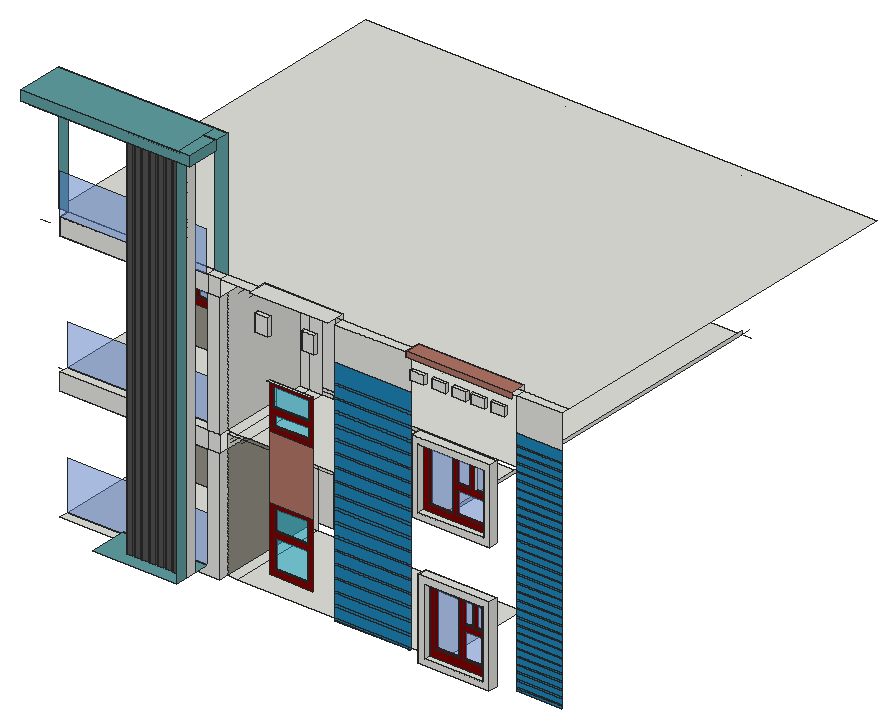
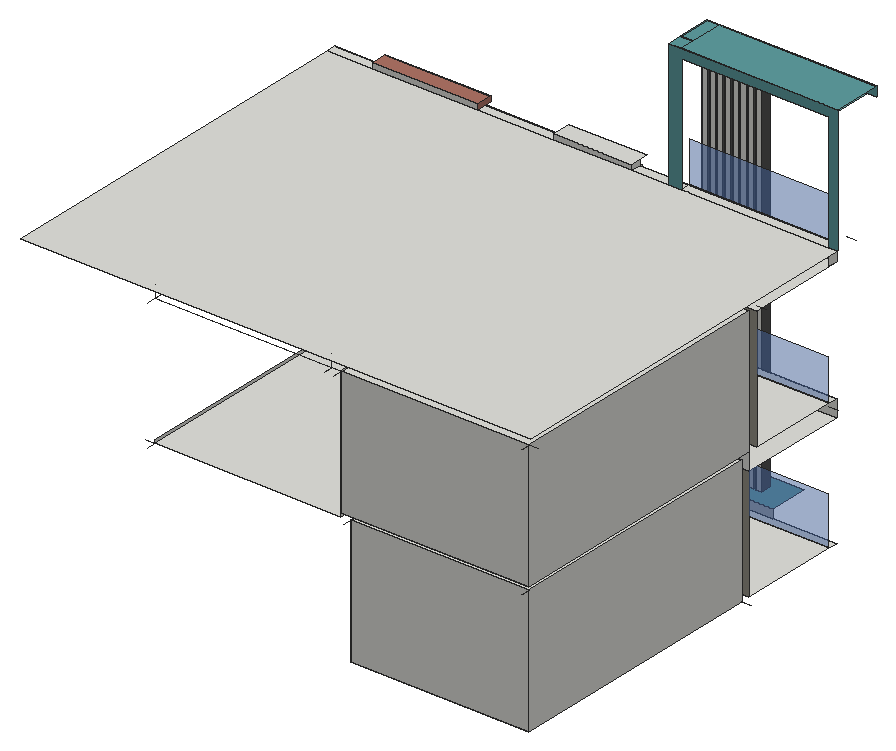
# SketchUp Ruby script. Lengths in inches.
U = 1.inch
M = Sketchup.active_model
def pt(a) = Geom::Point3d.new(a.map { |v| v * U })
def face(e, loops, mat)
  f = e.add_face(loops[0].map { |a| pt(a) })
  loops[1..].each { |l| e.add_face(l.map { |a| pt(a) }).erase! }
  f.material = f.back_material = mat if mat
  f
end
# faces: each face lists its corners as indices into pts; further lists are holes
def faces(e, pts, list, mat = nil) = list.each { |f| face(e, (f[0].is_a?(Array) ? f : [f]).map { |l| l.map { |i| pts[i] } }, mat) }
# xy, xz, yz: faces in a plane at the given z, y or x. An outline is a flat list of corners, or four numbers for a rectangle; further outlines are holes
def ring(l) = l.size == 4 ? [[l[0], l[1]], [l[2], l[1]], [l[2], l[3]], [l[0], l[3]]] : l.each_slice(2).to_a
def flat(e, list, mat, &to3) = list.each { |f| face(e, (f[0].is_a?(Array) ? f : [f]).map { |l| ring(l).map { |u, v| to3.(u, v) } }, mat) }
def xy(e, z, list, mat = nil) = flat(e, list, mat) { |x, y| [x, y, z] }
def xz(e, y, list, mat = nil) = flat(e, list, mat) { |x, z| [x, y, z] }
def yz(e, x, list, mat = nil) = flat(e, list, mat) { |y, z| [x, y, z] }
def lines(e, pts, list) = list.each { |a, b| e.add_line(pt(pts[a]), pt(pts[b])) }
# prism: a flat outline (further loops are holes) pulled along v
def prism(e, loops, v, mat = nil)
  f = face(e, loops, mat); d = Geom::Vector3d.new(v.map { |x| x * U })
  f.pushpull(f.normal.samedirection?(d) ? d.length : -d.length)
end
def box(e, o, s, mat = nil) = prism(e, [[o, [o[0] + s[0], o[1], o[2]], [o[0] + s[0], o[1] + s[1], o[2]], [o[0], o[1] + s[1], o[2]]]], [0, 0, s[2]], mat)
def at(x, y, z, deg = 0) = Geom::Transformation.translation(pt([x, y, z])) * Geom::Transformation.rotation(ORIGIN, Z_AXIS, deg.degrees)
def axes(o, x, y, z) = Geom::Transformation.new([*x, 0, *y, 0, *z, 0, *pt(o).to_a, 1])
def part(name) = M.definitions.add(name)
# library, detail: a bought-in or finely detailed component or shape, given as its bounding box
def library(name, o, s) = part(name).tap { |d| box(d.entities, o, s) }
def detail(e, o, s) = box(e.add_group.entities, o, s)
def put(e, d, t, mat = nil) = e.add_instance(d, t).tap { |i| i.material = mat if mat }
def group(e, t, mat = nil) = e.add_group.tap { |g| g.transformation = t; g.material = mat if mat }.entities
root = M.entities
M.materials.add("[0022_Maroon]").color = [128, 0, 0]
M.materials.add("[0081_CadetBlue]").color = [95, 158, 160]
M.materials.add("[0100_SteelBlue]").color = [29, 130, 180]
M.materials.add("[0135_DarkGray]").color = [81, 81, 81]
M.materials.add("[Formica Graystone]").color = [149, 146, 135]
M.materials.add("[Stone Flagstone Ashlar]").color = [175, 116, 102]
M.materials.add("[Translucent Glass Blue]").color = [100, 149, 237]
M.materials["[Translucent Glass Blue]"].alpha = 0.5
M.materials.add("[Translucent Glass Tinted]").color = [8, 201, 241]
M.materials["[Translucent Glass Tinted]"].alpha = 0.48
box(root,[9,148.25,428.75],[169.01,251.0625,120])
xy(root,428.75,[[9,36,160.01,45],[9,45,160.01,45,160.01,139.25,141.38,139.25,141.38,136.25,138.38,136.25,138.38,139.25,102.38,139.25,102.38,136.25,99.38,136.25,99.38,139.25,9,139.25],[160.01,45,170.26,139.25],[170.26,45,363.3125,139.25],[99.38,136.25,102.38,139.25],
  [138.38,136.25,141.38,139.25]])
xy(root,434.83,[[359.73,21,427.1,30]])
xy(root,437.26,[[[69.02,0,148.21,0,148.21,12,142.39,12,142.39,21.4,148.21,21.4,148.21,36,69.02,36],[98.52,12,98.52,21.4,104.33,21.4,104.33,12,105.83,12,105.83,21.4,111.64,21.4,111.64,12],[91.21,12,97.02,21.4],[127.77,12,133.58,21.4],[135.08,12,140.89,21.4]]],"[0081_CadetBlue]")
xy(root,437.3,[[113.14,12,118.96,21.4],[120.46,12,126.27,21.4]])
xy(root,440.83,[[365.73,21,421.1,27],[365.73,27,421.1,30]])
xy(root,447.86,[[371.08,27,393.35,30],[398.07,27,415.61,30]],"[0022_Maroon]")
xy(root,459.79,[[217.16,30,247.77,31.875]],"[0022_Maroon]")
xy(root,473.34,[[19,136.25,77.07,139.25]])
xy(root,473.35,[[398.07,27,415.61,30]],"[0022_Maroon]")
xy(root,477.84,[[398.07,27,406.84,30],[408.875,27,415.61,30]],"[0022_Maroon]")
xy(root,479.34,[[25,136.25,43.41,139.25],[48.03,136.25,71.07,139.25]],"[0022_Maroon]")
xy(root,486.74,[[217.16,30,247.77,31.875]],"[0022_Maroon]")
xy(root,492.12,[[217.16,30,247.77,32.25]],"[0022_Maroon]")
xy(root,498.84,[[371.08,27,393.35,30],[398.07,27,406.84,30],[408.875,27,415.61,30]],"[0022_Maroon]")
xy(root,504.21,[[365.73,21,421.1,27],[365.73,27,421.1,30]])
xy(root,504.65,[[48.03,136.25,71.07,139.25]],"[0022_Maroon]")
xy(root,508.1,[[48.03,136.25,71.07,139.25]],"[0022_Maroon]")
xy(root,510.21,[[359.73,21,427.1,30]])
xy(root,511.875,[[217.16,30,247.77,32.25]],"[0022_Maroon]")
xy(root,512.75,[[102.38,136.25,138.38,139.25]])
xy(root,515.75,[[99.38,136.25,141.38,139.25]])
xy(root,520.4,[[25,136.25,43.41,139.25],[48.03,136.25,71.07,139.25]],"[0022_Maroon]")
xy(root,526.4,[[19,136.25,77.07,139.25]])
xy(root,535.625,[[9,36,160.01,139.25]])
xy(root,548.75,[[160.01,45,170.26,139.25],[187.01,139.25,363.3125,399.3125]])
xy(root,551.75,[[9,36,160.01,45],[9,45,160.01,130.25],[160.01,45,170.26,130.25],[170.26,45,180.76,130.25],[180.76,45,363.3125,130.25],
  [9,139.25,187.01,399.3125]])
xy(root,556.6,[[353.5625,21,427.4375,30]])
xy(root,562.6,[[359.5625,21,421.4375,27]])
xy(root,568.2,[[365.03,27,387.7,30],[391.2,27,417.37,30]],"[0022_Maroon]")
xy(root,580.49,[[215.47,30,248.72,32.875]],"[0022_Maroon]")
xy(root,589.01,[[28.48,127.25,94.79,130.25]])
xy(root,590.47,[[391.2,27,417.37,30]],"[0022_Maroon]")
xy(root,591.16,[[215.47,30,248.72,32.875]],"[0022_Maroon]")
xy(root,595.01,[[34.48,127.25,61.63,130.25],[65.6,127.25,88.79,130.25]],"[0022_Maroon]")
xy(root,595.1,[[391.2,27,404.29,30],[408.3,27,417.37,30]],"[0022_Maroon]")
xy(root,596.41,[[215.47,32.3125,248.72,33.5]])
xy(root,596.47,[[215.47,30,248.72,32.3125]],"[0022_Maroon]")
xy(root,614.66,[[215.47,32.3125,248.72,33.5]])
xy(root,614.66,[[215.47,30,248.72,32.3125]],"[0022_Maroon]")
xy(root,616.91,[[365.03,27,387.7,30],[391.2,27,404.29,30],[408.3,27,417.37,30]],"[0022_Maroon]")
xy(root,619.47,[[211.91,27,253.16,30]])
xy(root,620.6,[[359.5625,21,421.4375,27]])
xy(root,626.6,[[353.5625,21,427.4375,30]])
xy(root,630.26,[[65.6,127.25,88.79,130.25]],"[0022_Maroon]")
xy(root,635.12,[[65.6,127.25,88.79,130.25]],"[0022_Maroon]")
xy(root,649.32,[[34.48,127.25,61.63,130.25],[65.6,127.25,88.79,130.25]],"[0022_Maroon]")
xy(root,655.32,[[28.48,127.25,94.79,130.25]])
xy(root,659.36,[[203.22,24,215.03,27],[246.9,24,258.72,27]])
xy(root,667.8125,[[9,36,160.01,130.25]])
xy(root,668.19,[[347.12,27,360.37,30],[367.68,27,380.93,30],[387.06,27,400.31,30],[404.68,27,417.93,30],[423.62,27,436.87,30]])
xy(root,671.75,[[9,139.25,187.01,399.3125]])
xy(root,675.93,[[203.22,24,215.03,27],[246.9,24,258.72,27]])
xy(root,676.37,[[347.12,27,360.37,30],[367.68,27,380.93,30],[387.06,27,400.31,30],[404.68,27,417.93,30],[423.62,27,436.87,30]])
xy(root,683.75,[[9,36,148.21,45],[148.21,36,160.01,45],[160.01,36,195.16,45],[269.35,36,341.01,45],[341.01,36,440.77,45],
  [440.77,36,483.5625,45],[0,45,483.5625,408.3125]])
xy(root,688.75,[[195.16,27,269.35,45]])
xy(root,688.75,[[341.01,30,440.77,45]],"[Stone Flagstone Ashlar]")
xy(root,794.55,[[91.21,12,97.02,21.4],[98.52,12,104.33,21.4],[105.83,12,111.64,21.4],[113.14,12,118.96,21.4],[120.46,12,126.27,21.4],
  [127.77,12,133.58,21.4],[135.08,12,140.89,21.4],[142.39,12,148.21,21.4]])
xy(root,794.55,[[[9,0,9,45,148.21,45,148.21,31.4375,160.01,31.4375,160.01,0,148.21,0,148.21,21.4,142.39,21.4,142.39,12,148.21,12,148.21,0],[91.21,12,97.02,21.4],[98.52,12,104.33,21.4],[105.83,12,111.64,21.4],[113.14,12,118.96,21.4],[120.46,12,126.27,21.4],[127.77,12,133.58,21.4],[135.08,12,140.89,21.4]]],"[0081_CadetBlue]")
xy(root,803.75,[[0,0,148.21,45],[148.21,0,160.01,31.4375],[148.21,31.4375,160.01,45]],"[0081_CadetBlue]")
xz(root,0,[[0,794.55,160.01,803.75]],"[0081_CadetBlue]")
xz(root,12,[[91.21,437.26,97.02,794.55],[98.52,437.26,104.33,794.55],[105.83,437.26,111.64,794.55],[127.77,437.26,133.58,794.55],[135.08,437.26,140.89,794.55],
  [142.39,437.26,148.21,794.55],[113.14,437.3,118.96,794.55],[120.46,437.3,126.27,794.55]],"[0135_DarkGray]")
xz(root,21,[[[359.73,434.83,427.1,510.21],[365.73,440.83,421.1,504.21]],[[353.5625,556.6,427.4375,626.6],[359.5625,562.6,421.4375,620.6]]])
xz(root,21.4,[[91.21,437.26,97.02,794.55],[98.52,437.26,104.33,794.55],[105.83,437.26,111.64,794.55],[127.77,437.26,133.58,794.55],[135.08,437.26,140.89,794.55],
  [142.39,437.26,148.21,794.55],[113.14,437.3,118.96,794.55],[120.46,437.3,126.27,794.55]])
xz(root,24,[[203.22,659.36,215.03,675.93],[246.9,659.36,258.72,675.93]])
xz(root,27,[[347.12,668.19,360.37,676.37],[367.68,668.19,380.93,676.37],[387.06,668.19,400.31,676.37],[404.68,668.19,417.93,676.37],[423.62,668.19,436.87,676.37]])
xz(root,27,[[[365.73,440.83,421.1,504.21],[371.08,447.86,393.35,498.84],[398.07,447.86,415.61,473.35],[398.07,477.84,406.84,498.84],[408.875,477.84,415.61,498.84]],[[359.5625,562.6,421.4375,620.6],[365.03,568.2,387.7,616.91],[391.2,568.2,417.37,590.47],[391.2,595.1,404.29,616.91],[408.3,595.1,417.37,616.91]]],"[0022_Maroon]")
xz(root,30,[[[359.73,434.83,427.1,510.21],[365.73,440.83,421.1,504.21]],[[365.73,440.83,421.1,504.21],[371.08,447.86,393.35,498.84],[398.07,447.86,415.61,473.35],[398.07,477.84,406.84,498.84],[408.875,477.84,415.61,498.84]]])
xz(root,30,[[[211.91,454.38,253.16,514.63],[217.16,459.79,247.77,486.74],[217.16,492.12,247.77,511.875]],[211.91,575.97,253.16,575.97,253.16,619.47,211.91,619.47,211.91,580.49,215.47,580.49,215.47,614.66,248.72,614.66,248.72,596.47,215.47,596.47,215.47,591.16,248.72,591.16,248.72,580.49,211.91,580.49]],"[0022_Maroon]")
xz(root,30,[[211.91,514.63,253.16,575.97],[341.01,683.75,440.77,688.75]],"[Stone Flagstone Ashlar]")
xz(root,30,[[371.08,447.86,393.35,498.84],[398.07,447.86,415.61,473.35],[398.07,477.84,406.84,498.84],[408.875,477.84,415.61,498.84],[365.03,568.2,387.7,616.91],
  [391.2,568.2,417.37,590.47],[391.2,595.1,404.29,616.91],[408.3,595.1,417.37,616.91]],"[Translucent Glass Blue]")
xz(root,31.4375,[[148.21,794.55,160.01,803.75]])
xz(root,31.875,[[217.16,459.79,247.77,486.74]],"[Translucent Glass Tinted]")
xz(root,32.25,[[217.16,492.12,247.77,511.875]],"[Translucent Glass Tinted]")
xz(root,32.3125,[[214.97,596.41,215.47,614.66],[215.47,596.41,248.72,596.47],[248.72,596.41,248.78,614.66],[215.47,614.66,248.72,614.72]])
xz(root,32.3125,[[215.47,596.47,248.72,614.66]],"[Translucent Glass Tinted]")
xz(root,32.875,[[215.47,580.49,248.72,591.16]],"[Translucent Glass Tinted]")
xz(root,33.5,[[215.47,596.41,248.72,614.66]])
xz(root,36,[[69.02,428.75,69.02,437.26,148.21,437.26,148.21,535.625,160.01,535.625,160.01,428.75],[9,535.625,148.21,551.75],[148.21,535.625,160.01,551.75],[148.21,551.75,160.01,667.8125],[269.35,651.87,341.01,683.75],
  [440.77,651.87,483.5625,683.75],[9,667.8125,148.21,683.75],[148.21,667.8125,160.01,683.75]])
xz(root,36,[[269.35,432.69,341.01,433.25],[269.35,433.25,341.01,434.71],[440.77,433.25,483.5625,435.22],[269.35,434.71,341.01,444.44],[440.77,435.22,483.5625,436.48],
  [440.77,436.48,483.5625,441.91],[440.77,441.91,483.5625,443.17],[440.77,443.17,483.5625,448.6],[269.35,444.44,341.01,446.46],[269.35,446.46,341.01,456.19],
  [440.77,448.6,483.5625,449.86],[440.77,449.86,483.5625,455.29],[440.77,455.29,483.5625,456.55],[269.35,456.19,341.01,458.21],[440.77,456.55,483.5625,461.97],
  [269.35,458.21,341.01,467.94],[440.77,461.97,483.5625,463.23],[440.77,463.23,483.5625,468.66],[269.35,467.94,341.01,469.96],[440.77,468.66,483.5625,469.92],
  [440.77,469.92,483.5625,475.35],[269.35,469.96,341.01,479.69],[440.77,475.35,483.5625,476.61],[440.77,476.61,483.5625,482.04],[269.35,479.69,341.01,481.71],
  [269.35,481.71,341.01,491.44],[440.77,482.04,483.5625,483.3],[440.77,483.3,483.5625,488.72],[440.77,488.72,483.5625,489.98],[440.77,489.98,483.5625,495.41],
  [269.35,491.44,341.01,493.46],[269.35,493.46,341.01,503.19],[440.77,495.41,483.5625,496.67],[440.77,496.67,483.5625,502.66],[440.77,502.66,483.5625,503.92],
  [269.35,503.19,341.01,505.21],[440.77,503.92,483.5625,509.91],[269.35,505.21,341.01,514.94],[440.77,509.91,483.5625,511.17],[440.77,511.17,483.5625,517.16],
  [269.35,514.94,341.01,516.96],[269.35,516.96,341.01,526.69],[440.77,517.16,483.5625,518.42],[440.77,518.42,483.5625,524.41],[440.77,524.41,483.5625,525.67],
  [440.77,525.67,483.5625,531.66],[269.35,526.69,341.01,528.71],[269.35,528.71,341.01,538.44],[440.77,531.66,483.5625,532.92],[440.77,532.92,483.5625,538.91],
  [269.35,538.44,341.01,540.46],[440.77,538.91,483.5625,540.17],[440.77,540.17,483.5625,546.16],[269.35,540.46,341.01,550.19],[440.77,546.16,483.5625,547.42],
  [440.77,547.42,483.5625,553.41],[269.35,550.19,341.01,552.21],[269.35,552.21,341.01,561.94],[440.77,553.41,483.5625,554.67],[440.77,554.67,483.5625,560.66],
  [440.77,560.66,483.5625,561.92],[440.77,561.92,483.5625,567.91],[269.35,561.94,341.01,563.96],[269.35,563.96,341.01,573.69],[440.77,567.91,483.5625,569.17],
  [440.77,569.17,483.5625,575.16],[269.35,573.69,341.01,575.71],[440.77,575.16,483.5625,576.42],[269.35,575.71,341.01,585.44],[440.77,576.42,483.5625,582.41],
  [440.77,582.41,483.5625,583.67],[440.77,583.67,483.5625,589.66],[269.35,585.44,341.01,587.46],[269.35,587.46,341.01,597.19],[440.77,589.66,483.5625,590.92],
  [440.77,590.92,483.5625,596.91],[440.77,596.91,483.5625,598.17],[269.35,597.19,341.01,599.21],[440.77,598.17,483.5625,604.16],[269.35,599.21,341.01,608.94],
  [440.77,604.16,483.5625,605.42],[440.77,605.42,483.5625,611.41],[269.35,608.94,341.01,610.96],[269.35,610.96,341.01,620.69],[440.77,611.41,483.5625,612.67],
  [440.77,612.67,483.5625,618.66],[440.77,618.66,483.5625,619.92],[440.77,619.92,483.5625,625.91],[269.35,620.69,341.01,622.71],[269.35,622.71,341.01,632.44],
  [440.77,625.91,483.5625,627.17],[440.77,627.17,483.5625,633.16],[269.35,632.44,341.01,634.46],[440.77,633.16,483.5625,634.42],[440.77,634.42,483.5625,640.41],
  [269.35,634.46,341.01,651.87],[440.77,640.41,483.5625,641.67],[440.77,641.67,483.5625,651.87]],"[0100_SteelBlue]")
xz(root,45,[[195.16,683.75,269.35,688.75],[341.01,683.75,440.77,688.75]])
xz(root,45,[[0,683.75,0,803.75,160.01,803.75,160.01,683.75,148.21,683.75,148.21,794.55,9,794.55,9,683.75]],"[0081_CadetBlue]")
xz(root,45,[[9,428.75,160.01,475.2],[9,551.75,160.01,590.95]],"[Translucent Glass Blue]")
xz(root,127.25,[[[28.48,589.01,94.79,655.32],[34.48,595.01,61.63,649.32],[65.6,595.01,88.79,630.26],[65.6,635.12,88.79,649.32]]],"[0022_Maroon]")
xz(root,130.25,[[160.01,551.75,170.26,671.75],[170.26,551.75,180.76,671.75],[[28.48,589.01,94.79,655.32],[34.48,595.01,61.63,649.32],[65.6,595.01,88.79,630.26],[65.6,635.12,88.79,649.32]]])
xz(root,130.25,[[[9,551.75,160.01,667.8125],[28.48,589.01,94.79,655.32]]],"[Formica Graystone]")
xz(root,130.25,[[34.48,595.01,61.63,649.32],[65.6,595.01,88.79,630.26],[65.6,635.12,88.79,649.32]],"[Translucent Glass Blue]")
xz(root,136.25,[[99.38,428.75,102.38,428.75,102.38,512.75,138.38,512.75,138.38,428.75,141.38,428.75,141.38,515.75,99.38,515.75]])
xz(root,136.25,[[[19,473.34,77.07,526.4],[25,479.34,43.41,520.4],[48.03,479.34,71.07,504.65],[48.03,508.1,71.07,520.4]]],"[0022_Maroon]")
xz(root,139.25,[[99.38,428.75,99.38,515.75,141.38,515.75,141.38,428.75,138.38,428.75,138.38,512.75,102.38,512.75,102.38,428.75],[102.38,428.75,138.38,512.75],[160.01,428.75,170.26,548.75],[9,535.625,160.01,535.625,160.01,548.75,187.01,548.75,187.01,551.75,9,551.75],[9,551.75,187.01,671.75]])
xz(root,139.25,[[[9,428.75,99.38,428.75,99.38,515.75,141.38,515.75,141.38,428.75,160.01,428.75,160.01,535.625,9,535.625],[19,473.34,77.07,526.4]]],"[Formica Graystone]")
xz(root,139.25,[[25,479.34,43.41,520.4],[48.03,479.34,71.07,504.65],[48.03,508.1,71.07,520.4]],"[Translucent Glass Blue]")
xz(root,399.3125,[[9,551.75,187.01,671.75]])
yz(root,9,[[139.25,551.75,399.3125,671.75],[36,667.8125,45,683.75]])
yz(root,19,[[136.25,473.34,139.25,526.4]])
yz(root,25,[[136.25,479.34,139.25,520.4]],"[0022_Maroon]")
yz(root,28.48,[[127.25,589.01,130.25,655.32]],"[0022_Maroon]")
yz(root,34.48,[[127.25,595.01,130.25,649.32]],"[0022_Maroon]")
yz(root,43.41,[[136.25,479.34,139.25,520.4]],"[0022_Maroon]")
yz(root,48.03,[[136.25,479.34,139.25,504.65],[136.25,508.1,139.25,520.4]],"[0022_Maroon]")
yz(root,61.63,[[127.25,595.01,130.25,649.32]],"[0022_Maroon]")
yz(root,65.6,[[127.25,595.01,130.25,630.26],[127.25,635.12,130.25,649.32]],"[0022_Maroon]")
yz(root,71.07,[[136.25,479.34,139.25,504.65],[136.25,508.1,139.25,520.4]],"[0022_Maroon]")
yz(root,77.07,[[136.25,473.34,139.25,526.4]])
yz(root,88.79,[[127.25,595.01,130.25,630.26],[127.25,635.12,130.25,649.32]],"[0022_Maroon]")
yz(root,91.21,[[12,437.26,21.4,794.55]],"[0135_DarkGray]")
yz(root,94.79,[[127.25,589.01,130.25,655.32]])
yz(root,97.02,[[12,437.26,21.4,794.55]],"[0135_DarkGray]")
yz(root,98.52,[[12,437.26,21.4,794.55]],"[0135_DarkGray]")
yz(root,99.38,[[136.25,428.75,139.25,515.75]])
yz(root,102.38,[[136.25,428.75,139.25,512.75]])
yz(root,104.33,[[12,437.26,21.4,794.55]],"[0135_DarkGray]")
yz(root,105.83,[[12,437.26,21.4,794.55]],"[0135_DarkGray]")
yz(root,111.64,[[12,437.26,21.4,794.55]],"[0135_DarkGray]")
yz(root,113.14,[[12,437.3,21.4,794.55]],"[0135_DarkGray]")
yz(root,118.96,[[12,437.3,21.4,794.55]],"[0135_DarkGray]")
yz(root,120.46,[[12,437.3,21.4,794.55]],"[0135_DarkGray]")
yz(root,126.27,[[12,437.3,21.4,794.55]],"[0135_DarkGray]")
yz(root,127.77,[[12,437.26,21.4,794.55]],"[0135_DarkGray]")
yz(root,133.58,[[12,437.26,21.4,794.55]],"[0135_DarkGray]")
yz(root,135.08,[[12,437.26,21.4,794.55]],"[0135_DarkGray]")
yz(root,138.38,[[136.25,428.75,139.25,512.75]])
yz(root,140.89,[[12,437.26,21.4,794.55]],"[0135_DarkGray]")
yz(root,141.38,[[136.25,428.75,139.25,515.75]])
yz(root,142.39,[[12,437.26,21.4,794.55]],"[0135_DarkGray]")
yz(root,148.21,[[12,437.26,21.4,794.55]])
yz(root,148.21,[[0,437.26,12,794.55]],"[0081_CadetBlue]")
yz(root,160.01,[[36,428.75,45,535.625],[45,535.625,139.25,548.75],[36,551.75,45,667.8125],[45,551.75,130.25,667.8125]])
yz(root,160.01,[[0,794.55,31.4375,803.75]],"[0081_CadetBlue]")
yz(root,160.01,[[45,428.75,139.25,535.625]],"[Formica Graystone]")
yz(root,187.01,[[139.25,548.75,399.3125,551.75],[139.25,551.75,399.3125,671.75]])
yz(root,195.16,[[36,683.75,45,688.75]])
yz(root,203.22,[[24,659.36,27,675.93]])
yz(root,215.03,[[24,659.36,27,675.93]])
yz(root,215.47,[[30,596.41,32.3125,596.47],[32.3125,596.41,33.5,614.66]])
yz(root,215.47,[[30,580.49,32.875,591.16],[30,596.47,32.3125,614.66]],"[0022_Maroon]")
yz(root,217.16,[[30,459.79,31.875,486.74],[30,492.12,32.25,511.875]],"[0022_Maroon]")
yz(root,246.9,[[24,659.36,27,675.93]])
yz(root,247.77,[[30,459.79,31.875,486.74],[30,492.12,32.25,511.875]],"[0022_Maroon]")
yz(root,248.72,[[32.3125,596.41,33.5,614.66]])
yz(root,248.72,[[30,580.49,32.875,591.16],[30,596.47,32.3125,614.66]],"[0022_Maroon]")
yz(root,258.72,[[24,659.36,27,675.93]])
yz(root,341.01,[[30,683.75,45,688.75]],"[Stone Flagstone Ashlar]")
yz(root,347.12,[[27,668.19,30,676.37]])
yz(root,353.5625,[[21,556.6,30,626.6]])
yz(root,359.5625,[[21,562.6,27,620.6]])
yz(root,359.73,[[21,434.83,30,510.21]])
yz(root,360.37,[[27,668.19,30,676.37]])
yz(root,363.3125,[[45,548.75,399.3125,551.75]])
yz(root,365.03,[[27,568.2,30,616.91]],"[0022_Maroon]")
yz(root,365.73,[[21,440.83,27,504.21],[27,440.83,30,504.21]])
yz(root,367.68,[[27,668.19,30,676.37]])
yz(root,371.08,[[27,447.86,30,498.84]],"[0022_Maroon]")
yz(root,380.93,[[27,668.19,30,676.37]])
yz(root,387.06,[[27,668.19,30,676.37]])
yz(root,387.7,[[27,568.2,30,616.91]],"[0022_Maroon]")
yz(root,391.2,[[27,568.2,30,590.47],[27,595.1,30,616.91]],"[0022_Maroon]")
yz(root,393.35,[[27,447.86,30,498.84]],"[0022_Maroon]")
yz(root,398.07,[[27,447.86,30,473.35],[27,477.84,30,498.84]],"[0022_Maroon]")
yz(root,400.31,[[27,668.19,30,676.37]])
yz(root,404.29,[[27,595.1,30,616.91]],"[0022_Maroon]")
yz(root,404.68,[[27,668.19,30,676.37]])
yz(root,406.84,[[27,477.84,30,498.84]],"[0022_Maroon]")
yz(root,408.3,[[27,595.1,30,616.91]])
yz(root,408.875,[[27,477.84,30,498.84]],"[0022_Maroon]")
yz(root,415.61,[[27,447.86,30,473.35],[27,477.84,30,498.84]],"[0022_Maroon]")
yz(root,417.37,[[27,568.2,30,590.47],[27,595.1,30,616.91]],"[0022_Maroon]")
yz(root,417.93,[[27,668.19,30,676.37]])
yz(root,421.1,[[21,440.83,27,504.21],[27,440.83,30,504.21]])
yz(root,421.4375,[[21,562.6,27,620.6]])
yz(root,423.62,[[27,668.19,30,676.37]])
yz(root,427.1,[[21,434.83,30,510.21]])
yz(root,427.4375,[[21,556.6,30,626.6]])
yz(root,436.87,[[27,668.19,30,676.37]])
p = [[9,36,683.75],[148.21,35.125,683.75],[148.21,35.125,722.625],[9,36,722.625],[9,148.25,428.75],[0,148.25,428.75],
  [178.01,399.3125,548.75],[178.01,408.3125,548.75],[9,399.3125,548.75],[9,408.3125,548.75],[363.3125,399.3125,548.75],[363.3125,408.3125,548.75],
  [372.3125,399.3125,548.75],[363.3125,45,551.75],[372.3125,45,551.75],[363.3125,45,671.75],[363.3125,130.25,671.75],[363.3125,399.3125,671.75],
  [363.3125,399.3125,683.75],[196.01,399.3125,671.75],[196.01,399.3125,683.75],[180.76,130.25,671.75],[9,399.3125,671.75],[0,399.3125,671.75],
  [9,130.25,671.75],[0,130.25,671.75],[187.01,399.3125,671.75],[187.01,408.3125,671.75],[9,408.3125,671.75],[196.01,408.3125,671.75],
  [363.3125,408.3125,671.75],[9,45,548.75],[0,45,548.75],[363.3125,45,548.75],[372.3125,45,548.75],[180.76,45,671.75],
  [170.26,45,548.75],[170.26,130.25,671.75],[170.26,45,671.75],[170.26,36,548.75],[363.3125,45,428.75],[363.3125,36,428.75],
  [180.76,45,551.75],[180.76,36,551.75],[170.26,45,551.75],[170.26,36,551.75],[9,24,683.75],[0,24,683.75],
  [248.72,30,596.41],[248.72,32.3125,596.41],[214.97,30,614.66],[214.97,32.3125,614.66],[214.97,30,596.41],[214.97,32.3125,596.41],
  [248.72,30,614.72],[248.72,32.3125,614.72],[215.47,30,614.72],[215.47,32.3125,614.72],[248.78,30,596.41],[248.78,32.3125,596.41],
  [248.78,30,614.66],[248.78,32.3125,614.66]]
faces(root,p,[[0,1,2,3]],"[Translucent Glass Blue]")
lines(root,p,[[4,5],[6,7],[8,9],[10,11],[10,12],[13,14],[15,16],[17,18],[19,20],[16,21],[22,23],[24,25],
  [26,27],[22,28],[19,29],[17,30],[31,32],[33,34],[21,35],[36,33],[17,19],[16,17],[19,26],[37,38],
  [36,39],[40,41],[42,43],[44,45],[46,47],[48,49],[50,51],[52,53],[54,55],[56,57],[58,59],[60,61]])
